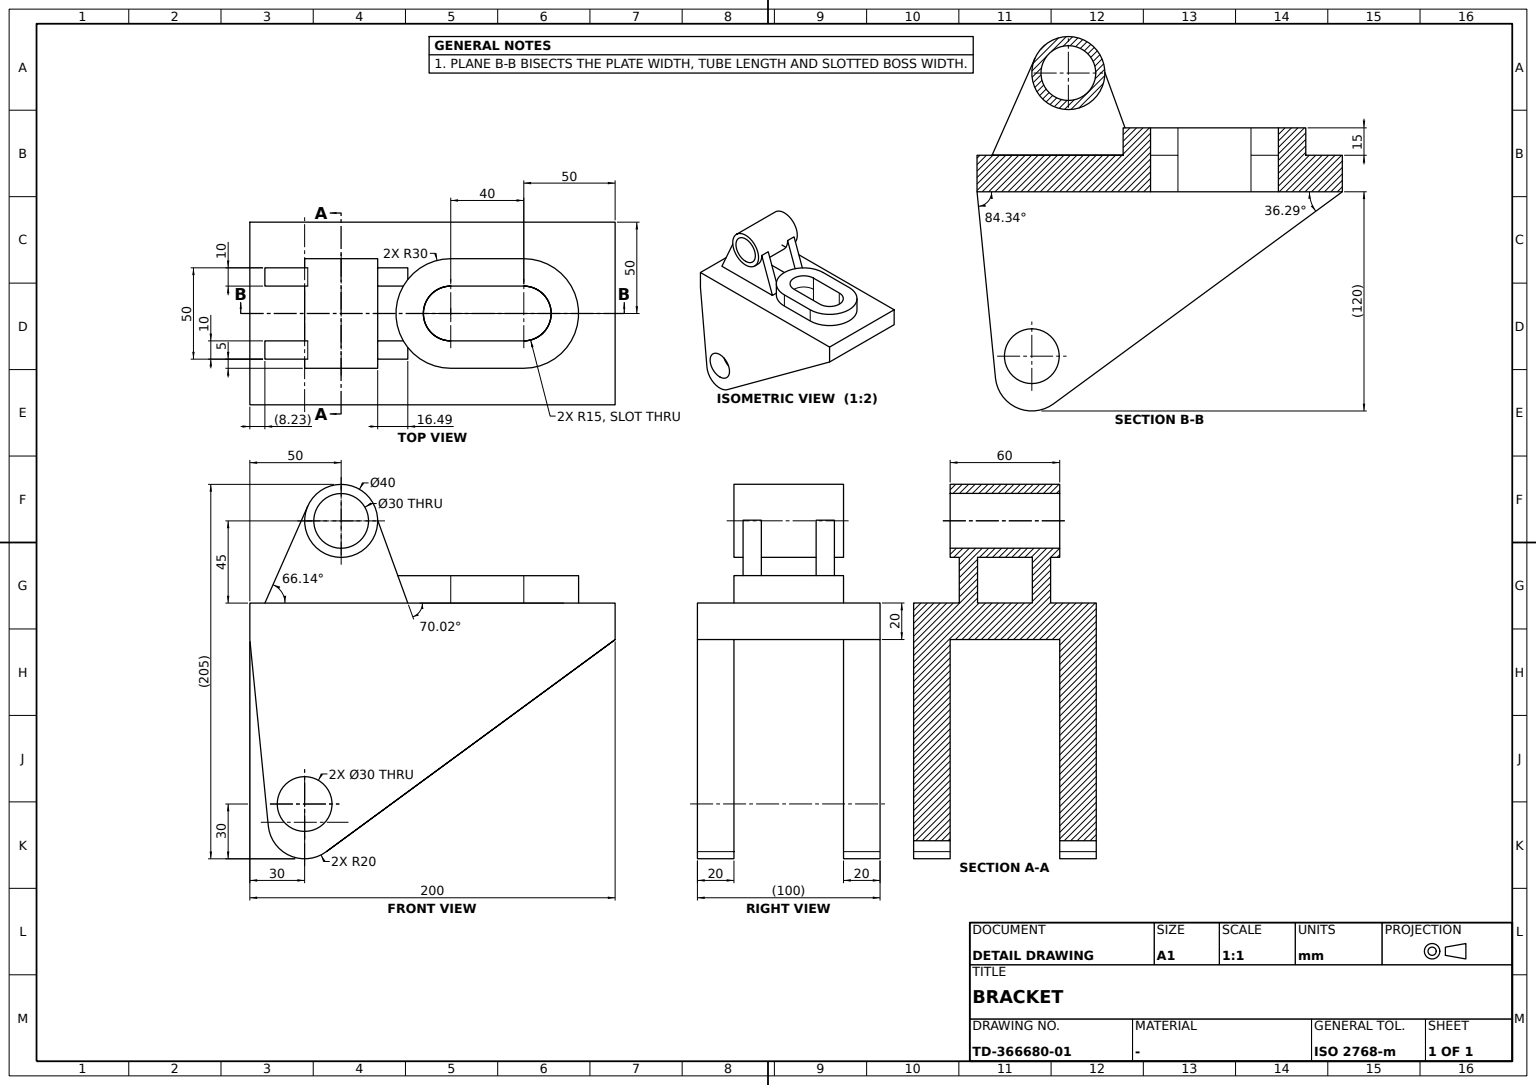
ISO-10303-21;
HEADER;
FILE_DESCRIPTION((''),'2;1');
FILE_NAME('','',(''),(''),'','','');
FILE_SCHEMA(('AUTOMOTIVE_DESIGN'));
ENDSEC;
DATA;
#1=APPLICATION_CONTEXT('');
#2=PRODUCT_CONTEXT('',#1,'mechanical');
#3=PRODUCT('','','',(#2));
#4=PRODUCT_DEFINITION_FORMATION('','',#3);
#5=PRODUCT_DEFINITION_CONTEXT('',#1,'design');
#6=PRODUCT_DEFINITION('','',#4,#5);
#7=PRODUCT_DEFINITION_SHAPE('','',#6);
#8=(LENGTH_UNIT()NAMED_UNIT(*)SI_UNIT(.MILLI.,.METRE.));
#9=(NAMED_UNIT(*)PLANE_ANGLE_UNIT()SI_UNIT($,.RADIAN.));
#10=(NAMED_UNIT(*)SI_UNIT($,.STERADIAN.)SOLID_ANGLE_UNIT());
#11=UNCERTAINTY_MEASURE_WITH_UNIT(LENGTH_MEASURE(0.005),#8,'distance_accuracy_value','');
#12=(GEOMETRIC_REPRESENTATION_CONTEXT(3)GLOBAL_UNCERTAINTY_ASSIGNED_CONTEXT((#11))GLOBAL_UNIT_ASSIGNED_CONTEXT((#8,#9,#10))REPRESENTATION_CONTEXT('',''));
#13=CARTESIAN_POINT('',(-48.163796,-50.,-136.121547));
#14=VERTEX_POINT('',#13);
#15=CARTESIAN_POINT('',(-48.163796,-30.,-136.121547));
#16=VERTEX_POINT('',#15);
#17=CARTESIAN_POINT('',(-48.163796,-40.,-136.121547));
#18=DIRECTION('',(0.,-1.,0.));
#19=VECTOR('',#18,1000.);
#20=LINE('',#17,#19);
#21=EDGE_CURVE('',#14,#16,#20,.F.);
#22=ORIENTED_EDGE('',*,*,#21,.F.);
#23=CARTESIAN_POINT('',(-79.902662,-50.,-121.970799));
#24=VERTEX_POINT('',#23);
#25=CARTESIAN_POINT('',(-60.,-50.,-120.));
#26=DIRECTION('',(0.,0.,-1.));
#27=AXIS2_PLACEMENT_3D('',#25,#18,#26);
#28=CIRCLE('',#27,20.);
#29=EDGE_CURVE('',#24,#14,#28,.T.);
#30=ORIENTED_EDGE('',*,*,#29,.F.);
#31=CARTESIAN_POINT('',(-79.902662,-30.,-121.970799));
#32=VERTEX_POINT('',#31);
#33=CARTESIAN_POINT('',(-79.902662,-40.,-121.970799));
#34=LINE('',#33,#19);
#35=EDGE_CURVE('',#24,#32,#34,.F.);
#36=ORIENTED_EDGE('',*,*,#35,.T.);
#37=CARTESIAN_POINT('',(-60.,-30.,-120.));
#38=AXIS2_PLACEMENT_3D('',#37,#18,#26);
#39=CIRCLE('',#38,20.);
#40=EDGE_CURVE('',#32,#16,#39,.T.);
#41=ORIENTED_EDGE('',*,*,#40,.T.);
#42=EDGE_LOOP('',(#22,#30,#36,#41));
#43=FACE_BOUND('',#42,.T.);
#44=CARTESIAN_POINT('',(-60.,-40.,-120.));
#45=DIRECTION('',(1.,0.,0.));
#46=AXIS2_PLACEMENT_3D('',#44,#18,#45);
#47=CYLINDRICAL_SURFACE('',#46,20.);
#48=ADVANCED_FACE('',(#43),#47,.T.);
#49=CARTESIAN_POINT('',(-5.980762,15.,6.781153));
#50=VERTEX_POINT('',#49);
#51=CARTESIAN_POINT('',(-20.002914,15.,45.34137));
#52=VERTEX_POINT('',#51);
#53=CARTESIAN_POINT('',(-3.514844,15.,0.));
#54=DIRECTION('',(-0.341748537,0.,0.939791433));
#55=VECTOR('',#54,1000.);
#56=LINE('',#53,#55);
#57=EDGE_CURVE('',#50,#52,#56,.T.);
#58=ORIENTED_EDGE('',*,*,#57,.F.);
#59=CARTESIAN_POINT('',(-3.514844,18.629335,0.));
#60=VERTEX_POINT('',#59);
#61=CARTESIAN_POINT('',(20.,0.,-64.664647));
#62=DIRECTION('',(-0.939791433,0.,-0.341748537));
#63=AXIS2_PLACEMENT_3D('',#61,#62,#54);
#64=ELLIPSE('',#63,87.783843,30.);
#65=EDGE_CURVE('',#50,#60,#64,.T.);
#66=ORIENTED_EDGE('',*,*,#65,.T.);
#67=CARTESIAN_POINT('',(-3.514844,25.,0.));
#68=VERTEX_POINT('',#67);
#69=CARTESIAN_POINT('',(-3.514844,0.,0.));
#70=LINE('',#69,#19);
#71=EDGE_CURVE('',#68,#60,#70,.T.);
#72=ORIENTED_EDGE('',*,*,#71,.F.);
#73=CARTESIAN_POINT('',(-20.002914,25.,45.34137));
#74=VERTEX_POINT('',#73);
#75=CARTESIAN_POINT('',(-3.104338,25.,-1.128871));
#76=LINE('',#75,#55);
#77=EDGE_CURVE('',#68,#74,#76,.T.);
#78=ORIENTED_EDGE('',*,*,#77,.T.);
#79=DIRECTION('',(0.,1.,0.));
#80=VECTOR('',#79,1000.);
#81=LINE('',#73,#80);
#82=EDGE_CURVE('',#74,#52,#81,.F.);
#83=ORIENTED_EDGE('',*,*,#82,.T.);
#84=EDGE_LOOP('',(#58,#66,#72,#78,#83));
#85=FACE_BOUND('',#84,.T.);
#86=CARTESIAN_POINT('',(-3.514844,-25.,0.));
#87=AXIS2_PLACEMENT_3D('',#86,#62,#54);
#88=PLANE('',#87);
#89=ADVANCED_FACE('',(#85),#88,.F.);
#90=CARTESIAN_POINT('',(20.,30.,15.));
#91=VERTEX_POINT('',#90);
#92=CARTESIAN_POINT('',(20.,-30.,15.));
#93=VERTEX_POINT('',#92);
#94=CARTESIAN_POINT('',(20.,0.,15.));
#95=DIRECTION('',(0.,0.,1.));
#96=AXIS2_PLACEMENT_3D('',#94,#95,#45);
#97=CIRCLE('',#96,30.);
#98=EDGE_CURVE('',#91,#93,#97,.T.);
#99=ORIENTED_EDGE('',*,*,#98,.F.);
#100=CARTESIAN_POINT('',(20.,30.,0.));
#101=VERTEX_POINT('',#100);
#102=CARTESIAN_POINT('',(20.,30.,7.5));
#103=VECTOR('',#95,1000.);
#104=LINE('',#102,#103);
#105=EDGE_CURVE('',#101,#91,#104,.T.);
#106=ORIENTED_EDGE('',*,*,#105,.F.);
#107=CARTESIAN_POINT('',(20.,0.,0.));
#108=AXIS2_PLACEMENT_3D('',#107,#95,#45);
#109=CIRCLE('',#108,30.);
#110=EDGE_CURVE('',#101,#60,#109,.T.);
#111=ORIENTED_EDGE('',*,*,#110,.T.);
#112=ORIENTED_EDGE('',*,*,#65,.F.);
#113=CARTESIAN_POINT('',(-5.980762,15.,0.));
#114=VERTEX_POINT('',#113);
#115=LINE('',#113,#103);
#116=EDGE_CURVE('',#114,#50,#115,.T.);
#117=ORIENTED_EDGE('',*,*,#116,.F.);
#118=CARTESIAN_POINT('',(-5.980762,-15.,0.));
#119=VERTEX_POINT('',#118);
#120=EDGE_CURVE('',#114,#119,#109,.T.);
#121=ORIENTED_EDGE('',*,*,#120,.T.);
#122=CARTESIAN_POINT('',(-5.980762,-15.,6.781153));
#123=VERTEX_POINT('',#122);
#124=LINE('',#118,#103);
#125=EDGE_CURVE('',#119,#123,#124,.T.);
#126=ORIENTED_EDGE('',*,*,#125,.T.);
#127=CARTESIAN_POINT('',(-3.514844,-18.629335,0.));
#128=VERTEX_POINT('',#127);
#129=EDGE_CURVE('',#123,#128,#64,.F.);
#130=ORIENTED_EDGE('',*,*,#129,.T.);
#131=CARTESIAN_POINT('',(20.,-30.,0.));
#132=VERTEX_POINT('',#131);
#133=EDGE_CURVE('',#128,#132,#109,.T.);
#134=ORIENTED_EDGE('',*,*,#133,.T.);
#135=CARTESIAN_POINT('',(20.,-30.,7.5));
#136=LINE('',#135,#103);
#137=EDGE_CURVE('',#132,#93,#136,.T.);
#138=ORIENTED_EDGE('',*,*,#137,.T.);
#139=EDGE_LOOP('',(#99,#106,#111,#112,#117,#121,#126,#130,#134,#138));
#140=FACE_BOUND('',#139,.T.);
#141=CARTESIAN_POINT('',(20.,0.,7.5));
#142=AXIS2_PLACEMENT_3D('',#141,#95,#45);
#143=CYLINDRICAL_SURFACE('',#142,30.);
#144=ADVANCED_FACE('',(#140),#143,.T.);
#145=CARTESIAN_POINT('',(-60.,30.,-95.));
#146=VERTEX_POINT('',#145);
#147=CARTESIAN_POINT('',(-60.,30.,-110.));
#148=AXIS2_PLACEMENT_3D('',#147,#79,#95);
#149=CIRCLE('',#148,15.);
#150=EDGE_CURVE('',#146,#146,#149,.T.);
#151=ORIENTED_EDGE('',*,*,#150,.T.);
#152=EDGE_LOOP('',(#151));
#153=FACE_BOUND('',#152,.T.);
#154=CARTESIAN_POINT('',(110.,30.,-20.));
#155=VERTEX_POINT('',#154);
#156=CARTESIAN_POINT('',(-90.,30.,-20.));
#157=VERTEX_POINT('',#156);
#158=CARTESIAN_POINT('',(0.,30.,-20.));
#159=DIRECTION('',(-1.,0.,0.));
#160=VECTOR('',#159,1000.);
#161=LINE('',#158,#160);
#162=EDGE_CURVE('',#155,#157,#161,.T.);
#163=ORIENTED_EDGE('',*,*,#162,.T.);
#164=CARTESIAN_POINT('',(-79.902662,30.,-121.970796));
#165=VERTEX_POINT('',#164);
#166=DIRECTION('',(0.098539929,0.,-0.995133098));
#167=VECTOR('',#166,1000.);
#168=LINE('',#156,#167);
#169=EDGE_CURVE('',#157,#165,#168,.T.);
#170=ORIENTED_EDGE('',*,*,#169,.T.);
#171=CARTESIAN_POINT('',(-48.163796,30.,-136.121547));
#172=VERTEX_POINT('',#171);
#173=CARTESIAN_POINT('',(-60.,30.,-120.));
#174=AXIS2_PLACEMENT_3D('',#173,#79,#95);
#175=CIRCLE('',#174,20.);
#176=EDGE_CURVE('',#172,#165,#175,.T.);
#177=ORIENTED_EDGE('',*,*,#176,.F.);
#178=DIRECTION('',(-0.806077344,0.,-0.591810202));
#179=VECTOR('',#178,1000.);
#180=LINE('',#154,#179);
#181=EDGE_CURVE('',#155,#172,#180,.T.);
#182=ORIENTED_EDGE('',*,*,#181,.F.);
#183=EDGE_LOOP('',(#163,#170,#177,#182));
#184=FACE_BOUND('',#183,.T.);
#185=CARTESIAN_POINT('',(0.,30.,0.));
#186=AXIS2_PLACEMENT_3D('',#185,#79,#159);
#187=PLANE('',#186);
#188=ADVANCED_FACE('',(#153,#184),#187,.F.);
#189=CARTESIAN_POINT('',(-58.291095,25.,53.089242));
#190=VERTEX_POINT('',#189);
#191=CARTESIAN_POINT('',(-40.,25.,45.));
#192=AXIS2_PLACEMENT_3D('',#191,#79,#95);
#193=CIRCLE('',#192,20.);
#194=EDGE_CURVE('',#74,#190,#193,.T.);
#195=ORIENTED_EDGE('',*,*,#194,.F.);
#196=ORIENTED_EDGE('',*,*,#77,.F.);
#197=CARTESIAN_POINT('',(-81.769829,25.,0.));
#198=VERTEX_POINT('',#197);
#199=CARTESIAN_POINT('',(0.,25.,0.));
#200=VECTOR('',#45,1000.);
#201=LINE('',#199,#200);
#202=EDGE_CURVE('',#198,#68,#201,.T.);
#203=ORIENTED_EDGE('',*,*,#202,.F.);
#204=CARTESIAN_POINT('',(-68.393135,25.,30.246885));
#205=DIRECTION('',(0.404462119,0.,0.914554752));
#206=VECTOR('',#205,1000.);
#207=LINE('',#204,#206);
#208=EDGE_CURVE('',#198,#190,#207,.T.);
#209=ORIENTED_EDGE('',*,*,#208,.T.);
#210=EDGE_LOOP('',(#195,#196,#203,#209));
#211=FACE_BOUND('',#210,.T.);
#212=AXIS2_PLACEMENT_3D('',#199,#79,#159);
#213=PLANE('',#212);
#214=ADVANCED_FACE('',(#211),#213,.T.);
#215=CARTESIAN_POINT('',(110.,-50.,-20.));
#216=VERTEX_POINT('',#215);
#217=DIRECTION('',(0.806077344,0.,0.591810202));
#218=VECTOR('',#217,1000.);
#219=LINE('',#215,#218);
#220=EDGE_CURVE('',#14,#216,#219,.T.);
#221=ORIENTED_EDGE('',*,*,#220,.F.);
#222=ORIENTED_EDGE('',*,*,#21,.T.);
#223=CARTESIAN_POINT('',(110.,-30.,-20.));
#224=VERTEX_POINT('',#223);
#225=LINE('',#223,#218);
#226=EDGE_CURVE('',#16,#224,#225,.T.);
#227=ORIENTED_EDGE('',*,*,#226,.T.);
#228=LINE('',#215,#80);
#229=EDGE_CURVE('',#216,#224,#228,.T.);
#230=ORIENTED_EDGE('',*,*,#229,.F.);
#231=EDGE_LOOP('',(#221,#222,#227,#230));
#232=FACE_BOUND('',#231,.T.);
#233=CARTESIAN_POINT('',(110.,50.,-20.));
#234=DIRECTION('',(-0.591810202,0.,0.806077344));
#235=AXIS2_PLACEMENT_3D('',#233,#234,#178);
#236=PLANE('',#235);
#237=ADVANCED_FACE('',(#232),#236,.F.);
#238=CARTESIAN_POINT('',(-40.,-30.,25.));
#239=VERTEX_POINT('',#238);
#240=CARTESIAN_POINT('',(-40.,-30.,45.));
#241=AXIS2_PLACEMENT_3D('',#240,#18,#26);
#242=CIRCLE('',#241,20.);
#243=EDGE_CURVE('',#239,#239,#242,.F.);
#244=ORIENTED_EDGE('',*,*,#243,.F.);
#245=EDGE_LOOP('',(#244));
#246=FACE_BOUND('',#245,.T.);
#247=CARTESIAN_POINT('',(-40.,-30.,30.));
#248=VERTEX_POINT('',#247);
#249=CIRCLE('',#241,15.);
#250=EDGE_CURVE('',#248,#248,#249,.F.);
#251=ORIENTED_EDGE('',*,*,#250,.T.);
#252=EDGE_LOOP('',(#251));
#253=FACE_BOUND('',#252,.T.);
#254=CARTESIAN_POINT('',(0.,-30.,0.));
#255=AXIS2_PLACEMENT_3D('',#254,#18,#45);
#256=PLANE('',#255);
#257=ADVANCED_FACE('',(#246,#253),#256,.T.);
#258=CARTESIAN_POINT('',(-81.769829,-25.,0.));
#259=VERTEX_POINT('',#258);
#260=CARTESIAN_POINT('',(-58.291095,-25.,53.089242));
#261=VERTEX_POINT('',#260);
#262=CARTESIAN_POINT('',(-68.393135,-25.,30.246885));
#263=LINE('',#262,#206);
#264=EDGE_CURVE('',#259,#261,#263,.T.);
#265=ORIENTED_EDGE('',*,*,#264,.F.);
#266=VERTEX_POINT('',#86);
#267=CARTESIAN_POINT('',(0.,-25.,0.));
#268=LINE('',#267,#200);
#269=EDGE_CURVE('',#259,#266,#268,.T.);
#270=ORIENTED_EDGE('',*,*,#269,.T.);
#271=CARTESIAN_POINT('',(-20.002914,-25.,45.34137));
#272=VERTEX_POINT('',#271);
#273=CARTESIAN_POINT('',(-3.104338,-25.,-1.128871));
#274=LINE('',#273,#55);
#275=EDGE_CURVE('',#266,#272,#274,.T.);
#276=ORIENTED_EDGE('',*,*,#275,.T.);
#277=CARTESIAN_POINT('',(-40.,-25.,45.));
#278=AXIS2_PLACEMENT_3D('',#277,#79,#95);
#279=CIRCLE('',#278,20.);
#280=EDGE_CURVE('',#272,#261,#279,.T.);
#281=ORIENTED_EDGE('',*,*,#280,.T.);
#282=EDGE_LOOP('',(#265,#270,#276,#281));
#283=FACE_BOUND('',#282,.T.);
#284=AXIS2_PLACEMENT_3D('',#267,#79,#159);
#285=PLANE('',#284);
#286=ADVANCED_FACE('',(#283),#285,.F.);
#287=CARTESIAN_POINT('',(60.,-15.,-20.));
#288=VERTEX_POINT('',#287);
#289=CARTESIAN_POINT('',(20.,-15.,-20.));
#290=VERTEX_POINT('',#289);
#291=CARTESIAN_POINT('',(0.,-15.,-20.));
#292=LINE('',#291,#160);
#293=EDGE_CURVE('',#288,#290,#292,.T.);
#294=ORIENTED_EDGE('',*,*,#293,.F.);
#295=CARTESIAN_POINT('',(60.,15.,-20.));
#296=VERTEX_POINT('',#295);
#297=CARTESIAN_POINT('',(62.356194,15.,-20.));
#298=CARTESIAN_POINT('',(64.712389,14.537362,-20.));
#299=CARTESIAN_POINT('',(66.947305,13.61163,-20.));
#300=CARTESIAN_POINT('',(70.933736,10.933736,-20.));
#301=CARTESIAN_POINT('',(73.61163,6.947305,-20.));
#302=CARTESIAN_POINT('',(74.537362,4.712389,-20.));
#303=CARTESIAN_POINT('',(75.462638,0.,-20.));
#304=CARTESIAN_POINT('',(74.537362,-4.712389,-20.));
#305=CARTESIAN_POINT('',(73.61163,-6.947305,-20.));
#306=CARTESIAN_POINT('',(70.933736,-10.933736,-20.));
#307=CARTESIAN_POINT('',(66.947305,-13.61163,-20.));
#308=CARTESIAN_POINT('',(64.712389,-14.537362,-20.));
#309=CARTESIAN_POINT('',(62.356194,-15.,-20.));
#310=B_SPLINE_CURVE_WITH_KNOTS('',5,(#295,#297,#298,#299,#300,#301,#302,#303,#304,#305,#306,#307,#308,#309,#287),.UNSPECIFIED.,.F.,.F.,(6,3,3,3,6),(0.,0.012,0.024,0.036,0.048),.UNSPECIFIED.);
#311=EDGE_CURVE('',#296,#288,#310,.T.);
#312=ORIENTED_EDGE('',*,*,#311,.F.);
#313=CARTESIAN_POINT('',(20.,15.,-20.));
#314=VERTEX_POINT('',#313);
#315=CARTESIAN_POINT('',(0.,15.,-20.));
#316=LINE('',#315,#200);
#317=EDGE_CURVE('',#314,#296,#316,.T.);
#318=ORIENTED_EDGE('',*,*,#317,.F.);
#319=CARTESIAN_POINT('',(17.643806,-15.,-20.));
#320=CARTESIAN_POINT('',(15.287611,-14.537362,-20.));
#321=CARTESIAN_POINT('',(13.052695,-13.61163,-20.));
#322=CARTESIAN_POINT('',(9.066264,-10.933736,-20.));
#323=CARTESIAN_POINT('',(6.38837,-6.947305,-20.));
#324=CARTESIAN_POINT('',(5.462638,-4.712389,-20.));
#325=CARTESIAN_POINT('',(4.537362,0.,-20.));
#326=CARTESIAN_POINT('',(5.462638,4.712389,-20.));
#327=CARTESIAN_POINT('',(6.38837,6.947305,-20.));
#328=CARTESIAN_POINT('',(9.066264,10.933736,-20.));
#329=CARTESIAN_POINT('',(13.052695,13.61163,-20.));
#330=CARTESIAN_POINT('',(15.287611,14.537362,-20.));
#331=CARTESIAN_POINT('',(17.643806,15.,-20.));
#332=B_SPLINE_CURVE_WITH_KNOTS('',5,(#289,#319,#320,#321,#322,#323,#324,#325,#326,#327,#328,#329,#330,#331,#313),.UNSPECIFIED.,.F.,.F.,(6,3,3,3,6),(0.,0.012,0.024,0.036,0.048),.UNSPECIFIED.);
#333=EDGE_CURVE('',#290,#314,#332,.T.);
#334=ORIENTED_EDGE('',*,*,#333,.F.);
#335=EDGE_LOOP('',(#294,#312,#318,#334));
#336=FACE_BOUND('',#335,.T.);
#337=ORIENTED_EDGE('',*,*,#162,.F.);
#338=EDGE_CURVE('',#224,#155,#228,.T.);
#339=ORIENTED_EDGE('',*,*,#338,.F.);
#340=CARTESIAN_POINT('',(-90.,-30.,-20.));
#341=VERTEX_POINT('',#340);
#342=CARTESIAN_POINT('',(0.,-30.,-20.));
#343=LINE('',#342,#200);
#344=EDGE_CURVE('',#341,#224,#343,.T.);
#345=ORIENTED_EDGE('',*,*,#344,.F.);
#346=CARTESIAN_POINT('',(-90.,50.,-20.));
#347=LINE('',#346,#19);
#348=EDGE_CURVE('',#157,#341,#347,.T.);
#349=ORIENTED_EDGE('',*,*,#348,.F.);
#350=EDGE_LOOP('',(#337,#339,#345,#349));
#351=FACE_BOUND('',#350,.T.);
#352=CARTESIAN_POINT('',(0.,0.,-20.));
#353=AXIS2_PLACEMENT_3D('',#352,#95,#45);
#354=PLANE('',#353);
#355=ADVANCED_FACE('',(#336,#351),#354,.F.);
#356=VERTEX_POINT('',#233);
#357=LINE('',#233,#19);
#358=EDGE_CURVE('',#356,#155,#357,.T.);
#359=ORIENTED_EDGE('',*,*,#358,.T.);
#360=ORIENTED_EDGE('',*,*,#181,.T.);
#361=CARTESIAN_POINT('',(-48.163794,50.,-136.121545));
#362=VERTEX_POINT('',#361);
#363=EDGE_CURVE('',#362,#172,#20,.T.);
#364=ORIENTED_EDGE('',*,*,#363,.F.);
#365=LINE('',#233,#179);
#366=EDGE_CURVE('',#356,#362,#365,.T.);
#367=ORIENTED_EDGE('',*,*,#366,.F.);
#368=EDGE_LOOP('',(#359,#360,#364,#367));
#369=FACE_BOUND('',#368,.T.);
#370=ADVANCED_FACE('',(#369),#236,.F.);
#371=CARTESIAN_POINT('',(-60.,-30.,-125.));
#372=VERTEX_POINT('',#371);
#373=CARTESIAN_POINT('',(-60.,-30.,-110.));
#374=AXIS2_PLACEMENT_3D('',#373,#18,#26);
#375=CIRCLE('',#374,15.);
#376=EDGE_CURVE('',#372,#372,#375,.T.);
#377=ORIENTED_EDGE('',*,*,#376,.T.);
#378=EDGE_LOOP('',(#377));
#379=FACE_BOUND('',#378,.T.);
#380=ORIENTED_EDGE('',*,*,#226,.F.);
#381=ORIENTED_EDGE('',*,*,#40,.F.);
#382=CARTESIAN_POINT('',(-91.087296,-30.,-9.019633));
#383=LINE('',#382,#167);
#384=EDGE_CURVE('',#341,#32,#383,.T.);
#385=ORIENTED_EDGE('',*,*,#384,.F.);
#386=ORIENTED_EDGE('',*,*,#344,.T.);
#387=EDGE_LOOP('',(#380,#381,#385,#386));
#388=FACE_BOUND('',#387,.T.);
#389=ADVANCED_FACE('',(#379,#388),#256,.F.);
#390=CARTESIAN_POINT('',(20.,-15.,0.));
#391=VERTEX_POINT('',#390);
#392=LINE('',#390,#103);
#393=EDGE_CURVE('',#391,#290,#392,.F.);
#394=ORIENTED_EDGE('',*,*,#393,.T.);
#395=ORIENTED_EDGE('',*,*,#333,.T.);
#396=CARTESIAN_POINT('',(20.,15.,0.));
#397=VERTEX_POINT('',#396);
#398=LINE('',#396,#103);
#399=EDGE_CURVE('',#397,#314,#398,.F.);
#400=ORIENTED_EDGE('',*,*,#399,.F.);
#401=CARTESIAN_POINT('',(16.073009,-15.,0.));
#402=CARTESIAN_POINT('',(8.250292,-11.754174,0.));
#403=CARTESIAN_POINT('',(3.374854,0.,0.));
#404=CARTESIAN_POINT('',(8.250292,11.754174,0.));
#405=CARTESIAN_POINT('',(16.073009,15.,0.));
#406=B_SPLINE_CURVE_WITH_KNOTS('',3,(#390,#401,#402,#403,#404,#405,#396),.UNSPECIFIED.,.F.,.F.,(4,1,1,1,4),(23.561944902,35.342917353,47.123889804,58.904862255,70.685834706),.UNSPECIFIED.);
#407=EDGE_CURVE('',#397,#391,#406,.F.);
#408=ORIENTED_EDGE('',*,*,#407,.T.);
#409=EDGE_LOOP('',(#394,#395,#400,#408));
#410=FACE_BOUND('',#409,.T.);
#411=CARTESIAN_POINT('',(16.073009,-15.,-20.));
#412=CARTESIAN_POINT('',(8.250292,-11.754174,-20.));
#413=CARTESIAN_POINT('',(3.374854,0.,-20.));
#414=CARTESIAN_POINT('',(8.250292,11.754174,-20.));
#415=CARTESIAN_POINT('',(16.073009,15.,-20.));
#416=B_SPLINE_SURFACE_WITH_KNOTS('',3,1,((#390,#289),(#401,#411),(#402,#412),(#403,#413),(#404,#414),(#405,#415),(#396,#313)),.SURF_OF_LINEAR_EXTRUSION.,.F.,.F.,.F.,(4,1,1,1,4),(2,2),(0.,0.012,0.024,0.036,0.048),(0.,1.),.UNSPECIFIED.);
#417=ADVANCED_FACE('',(#410),#416,.F.);
#418=ORIENTED_EDGE('',*,*,#243,.T.);
#419=EDGE_LOOP('',(#418));
#420=FACE_BOUND('',#419,.T.);
#421=CARTESIAN_POINT('',(-40.,30.,65.));
#422=VERTEX_POINT('',#421);
#423=CARTESIAN_POINT('',(-40.,30.,45.));
#424=AXIS2_PLACEMENT_3D('',#423,#79,#95);
#425=CIRCLE('',#424,20.);
#426=EDGE_CURVE('',#422,#422,#425,.T.);
#427=ORIENTED_EDGE('',*,*,#426,.F.);
#428=EDGE_LOOP('',(#427));
#429=FACE_BOUND('',#428,.T.);
#430=ORIENTED_EDGE('',*,*,#280,.F.);
#431=CARTESIAN_POINT('',(-20.002914,-15.,45.34137));
#432=VERTEX_POINT('',#431);
#433=LINE('',#271,#80);
#434=EDGE_CURVE('',#272,#432,#433,.T.);
#435=ORIENTED_EDGE('',*,*,#434,.T.);
#436=CARTESIAN_POINT('',(-58.291095,-15.,53.089242));
#437=VERTEX_POINT('',#436);
#438=CARTESIAN_POINT('',(-40.,-15.,45.));
#439=AXIS2_PLACEMENT_3D('',#438,#79,#95);
#440=CIRCLE('',#439,20.);
#441=EDGE_CURVE('',#432,#437,#440,.T.);
#442=ORIENTED_EDGE('',*,*,#441,.T.);
#443=CARTESIAN_POINT('',(-58.291095,0.,53.089242));
#444=LINE('',#443,#80);
#445=EDGE_CURVE('',#261,#437,#444,.T.);
#446=ORIENTED_EDGE('',*,*,#445,.F.);
#447=EDGE_LOOP('',(#430,#435,#442,#446));
#448=FACE_BOUND('',#447,.T.);
#449=ORIENTED_EDGE('',*,*,#194,.T.);
#450=CARTESIAN_POINT('',(-58.291095,15.,53.089242));
#451=VERTEX_POINT('',#450);
#452=EDGE_CURVE('',#190,#451,#444,.F.);
#453=ORIENTED_EDGE('',*,*,#452,.T.);
#454=CARTESIAN_POINT('',(-40.,15.,45.));
#455=AXIS2_PLACEMENT_3D('',#454,#18,#26);
#456=CIRCLE('',#455,20.);
#457=EDGE_CURVE('',#451,#52,#456,.T.);
#458=ORIENTED_EDGE('',*,*,#457,.T.);
#459=ORIENTED_EDGE('',*,*,#82,.F.);
#460=EDGE_LOOP('',(#449,#453,#458,#459));
#461=FACE_BOUND('',#460,.T.);
#462=CARTESIAN_POINT('',(-40.,0.,45.));
#463=AXIS2_PLACEMENT_3D('',#462,#79,#159);
#464=CYLINDRICAL_SURFACE('',#463,20.);
#465=ADVANCED_FACE('',(#420,#429,#448,#461),#464,.T.);
#466=VERTEX_POINT('',#346);
#467=EDGE_CURVE('',#466,#157,#347,.T.);
#468=ORIENTED_EDGE('',*,*,#467,.F.);
#469=CARTESIAN_POINT('',(-79.902662,50.,-121.970799));
#470=VERTEX_POINT('',#469);
#471=LINE('',#346,#167);
#472=EDGE_CURVE('',#466,#470,#471,.T.);
#473=ORIENTED_EDGE('',*,*,#472,.T.);
#474=EDGE_CURVE('',#470,#165,#34,.T.);
#475=ORIENTED_EDGE('',*,*,#474,.T.);
#476=ORIENTED_EDGE('',*,*,#169,.F.);
#477=EDGE_LOOP('',(#468,#473,#475,#476));
#478=FACE_BOUND('',#477,.T.);
#479=DIRECTION('',(-0.995133098,0.,-0.098539929));
#480=AXIS2_PLACEMENT_3D('',#346,#479,#166);
#481=PLANE('',#480);
#482=ADVANCED_FACE('',(#478),#481,.T.);
#483=CARTESIAN_POINT('',(-60.,50.,-95.));
#484=VERTEX_POINT('',#483);
#485=CARTESIAN_POINT('',(-60.,50.,-110.));
#486=AXIS2_PLACEMENT_3D('',#485,#79,#95);
#487=CIRCLE('',#486,15.);
#488=EDGE_CURVE('',#484,#484,#487,.T.);
#489=ORIENTED_EDGE('',*,*,#488,.T.);
#490=EDGE_LOOP('',(#489));
#491=FACE_BOUND('',#490,.T.);
#492=ORIENTED_EDGE('',*,*,#150,.F.);
#493=EDGE_LOOP('',(#492));
#494=FACE_BOUND('',#493,.T.);
#495=CARTESIAN_POINT('',(-60.,-0.66,-110.));
#496=AXIS2_PLACEMENT_3D('',#495,#79,#159);
#497=CYLINDRICAL_SURFACE('',#496,15.);
#498=ADVANCED_FACE('',(#491,#494),#497,.F.);
#499=CARTESIAN_POINT('',(60.,30.,0.));
#500=VERTEX_POINT('',#499);
#501=LINE('',#185,#200);
#502=EDGE_CURVE('',#101,#500,#501,.T.);
#503=ORIENTED_EDGE('',*,*,#502,.F.);
#504=ORIENTED_EDGE('',*,*,#105,.T.);
#505=CARTESIAN_POINT('',(60.,30.,15.));
#506=VERTEX_POINT('',#505);
#507=CARTESIAN_POINT('',(0.,30.,15.));
#508=LINE('',#507,#200);
#509=EDGE_CURVE('',#91,#506,#508,.T.);
#510=ORIENTED_EDGE('',*,*,#509,.T.);
#511=CARTESIAN_POINT('',(60.,30.,7.5));
#512=LINE('',#511,#103);
#513=EDGE_CURVE('',#500,#506,#512,.T.);
#514=ORIENTED_EDGE('',*,*,#513,.F.);
#515=EDGE_LOOP('',(#503,#504,#510,#514));
#516=FACE_BOUND('',#515,.T.);
#517=ADVANCED_FACE('',(#516),#187,.T.);
#518=CARTESIAN_POINT('',(60.,-15.,15.));
#519=VERTEX_POINT('',#518);
#520=CARTESIAN_POINT('',(60.,15.,15.));
#521=VERTEX_POINT('',#520);
#522=CARTESIAN_POINT('',(60.,0.,15.));
#523=AXIS2_PLACEMENT_3D('',#522,#95,#45);
#524=CIRCLE('',#523,15.);
#525=EDGE_CURVE('',#519,#521,#524,.T.);
#526=ORIENTED_EDGE('',*,*,#525,.T.);
#527=CARTESIAN_POINT('',(60.,15.,0.));
#528=VERTEX_POINT('',#527);
#529=CARTESIAN_POINT('',(60.,15.,7.5));
#530=LINE('',#529,#103);
#531=EDGE_CURVE('',#528,#521,#530,.T.);
#532=ORIENTED_EDGE('',*,*,#531,.F.);
#533=CARTESIAN_POINT('',(60.,-15.,0.));
#534=VERTEX_POINT('',#533);
#535=CARTESIAN_POINT('',(63.926991,15.,0.));
#536=CARTESIAN_POINT('',(71.749708,11.754174,0.));
#537=CARTESIAN_POINT('',(76.625146,0.,0.));
#538=CARTESIAN_POINT('',(71.749708,-11.754174,0.));
#539=CARTESIAN_POINT('',(63.926991,-15.,0.));
#540=B_SPLINE_CURVE_WITH_KNOTS('',3,(#527,#535,#536,#537,#538,#539,#533),.UNSPECIFIED.,.F.,.F.,(4,1,1,1,4),(70.685834706,82.466807157,94.247779608,106.028752059,117.80972451),.UNSPECIFIED.);
#541=EDGE_CURVE('',#528,#534,#540,.T.);
#542=ORIENTED_EDGE('',*,*,#541,.T.);
#543=CARTESIAN_POINT('',(60.,-15.,7.5));
#544=LINE('',#543,#103);
#545=EDGE_CURVE('',#534,#519,#544,.T.);
#546=ORIENTED_EDGE('',*,*,#545,.T.);
#547=EDGE_LOOP('',(#526,#532,#542,#546));
#548=FACE_BOUND('',#547,.T.);
#549=CARTESIAN_POINT('',(60.,0.,7.5));
#550=AXIS2_PLACEMENT_3D('',#549,#95,#45);
#551=CYLINDRICAL_SURFACE('',#550,15.);
#552=ADVANCED_FACE('',(#548),#551,.F.);
#553=ORIENTED_EDGE('',*,*,#317,.T.);
#554=LINE('',#527,#103);
#555=EDGE_CURVE('',#528,#296,#554,.F.);
#556=ORIENTED_EDGE('',*,*,#555,.F.);
#557=ORIENTED_EDGE('',*,*,#531,.T.);
#558=CARTESIAN_POINT('',(20.,15.,15.));
#559=VERTEX_POINT('',#558);
#560=CARTESIAN_POINT('',(0.,15.,15.));
#561=LINE('',#560,#200);
#562=EDGE_CURVE('',#559,#521,#561,.T.);
#563=ORIENTED_EDGE('',*,*,#562,.F.);
#564=CARTESIAN_POINT('',(20.,15.,7.5));
#565=LINE('',#564,#103);
#566=EDGE_CURVE('',#397,#559,#565,.T.);
#567=ORIENTED_EDGE('',*,*,#566,.F.);
#568=ORIENTED_EDGE('',*,*,#399,.T.);
#569=EDGE_LOOP('',(#553,#556,#557,#563,#567,#568));
#570=FACE_BOUND('',#569,.T.);
#571=AXIS2_PLACEMENT_3D('',#396,#18,#45);
#572=PLANE('',#571);
#573=ADVANCED_FACE('',(#570),#572,.T.);
#574=ORIENTED_EDGE('',*,*,#376,.F.);
#575=EDGE_LOOP('',(#574));
#576=FACE_BOUND('',#575,.T.);
#577=CARTESIAN_POINT('',(-60.,-50.,-125.));
#578=VERTEX_POINT('',#577);
#579=CARTESIAN_POINT('',(-60.,-50.,-110.));
#580=AXIS2_PLACEMENT_3D('',#579,#18,#26);
#581=CIRCLE('',#580,15.);
#582=EDGE_CURVE('',#578,#578,#581,.T.);
#583=ORIENTED_EDGE('',*,*,#582,.T.);
#584=EDGE_LOOP('',(#583));
#585=FACE_BOUND('',#584,.T.);
#586=ADVANCED_FACE('',(#576,#585),#497,.F.);
#587=ORIENTED_EDGE('',*,*,#566,.T.);
#588=CARTESIAN_POINT('',(20.,-15.,15.));
#589=VERTEX_POINT('',#588);
#590=CIRCLE('',#96,15.);
#591=EDGE_CURVE('',#559,#589,#590,.T.);
#592=ORIENTED_EDGE('',*,*,#591,.T.);
#593=CARTESIAN_POINT('',(20.,-15.,7.5));
#594=LINE('',#593,#103);
#595=EDGE_CURVE('',#391,#589,#594,.T.);
#596=ORIENTED_EDGE('',*,*,#595,.F.);
#597=ORIENTED_EDGE('',*,*,#407,.F.);
#598=EDGE_LOOP('',(#587,#592,#596,#597));
#599=FACE_BOUND('',#598,.T.);
#600=CYLINDRICAL_SURFACE('',#142,15.);
#601=ADVANCED_FACE('',(#599),#600,.F.);
#602=ORIENTED_EDGE('',*,*,#98,.T.);
#603=CARTESIAN_POINT('',(60.,-30.,15.));
#604=VERTEX_POINT('',#603);
#605=CARTESIAN_POINT('',(0.,-30.,15.));
#606=LINE('',#605,#160);
#607=EDGE_CURVE('',#604,#93,#606,.T.);
#608=ORIENTED_EDGE('',*,*,#607,.F.);
#609=CIRCLE('',#523,30.);
#610=EDGE_CURVE('',#604,#506,#609,.T.);
#611=ORIENTED_EDGE('',*,*,#610,.T.);
#612=ORIENTED_EDGE('',*,*,#509,.F.);
#613=EDGE_LOOP('',(#602,#608,#611,#612));
#614=FACE_BOUND('',#613,.T.);
#615=ORIENTED_EDGE('',*,*,#591,.F.);
#616=ORIENTED_EDGE('',*,*,#562,.T.);
#617=ORIENTED_EDGE('',*,*,#525,.F.);
#618=CARTESIAN_POINT('',(0.,-15.,15.));
#619=LINE('',#618,#160);
#620=EDGE_CURVE('',#519,#589,#619,.T.);
#621=ORIENTED_EDGE('',*,*,#620,.T.);
#622=EDGE_LOOP('',(#615,#616,#617,#621));
#623=FACE_BOUND('',#622,.T.);
#624=CARTESIAN_POINT('',(0.,0.,15.));
#625=AXIS2_PLACEMENT_3D('',#624,#95,#45);
#626=PLANE('',#625);
#627=ADVANCED_FACE('',(#614,#623),#626,.T.);
#628=CARTESIAN_POINT('',(-60.,50.,-120.));
#629=AXIS2_PLACEMENT_3D('',#628,#79,#95);
#630=CIRCLE('',#629,20.);
#631=EDGE_CURVE('',#362,#470,#630,.T.);
#632=ORIENTED_EDGE('',*,*,#631,.F.);
#633=ORIENTED_EDGE('',*,*,#363,.T.);
#634=ORIENTED_EDGE('',*,*,#176,.T.);
#635=ORIENTED_EDGE('',*,*,#474,.F.);
#636=EDGE_LOOP('',(#632,#633,#634,#635));
#637=FACE_BOUND('',#636,.T.);
#638=ADVANCED_FACE('',(#637),#47,.T.);
#639=CARTESIAN_POINT('',(-81.769829,-15.,0.));
#640=VERTEX_POINT('',#639);
#641=LINE('',#533,#200);
#642=EDGE_CURVE('',#640,#119,#641,.T.);
#643=ORIENTED_EDGE('',*,*,#642,.T.);
#644=ORIENTED_EDGE('',*,*,#120,.F.);
#645=CARTESIAN_POINT('',(-81.769829,15.,0.));
#646=VERTEX_POINT('',#645);
#647=CARTESIAN_POINT('',(0.,15.,0.));
#648=LINE('',#647,#200);
#649=EDGE_CURVE('',#646,#114,#648,.T.);
#650=ORIENTED_EDGE('',*,*,#649,.F.);
#651=CARTESIAN_POINT('',(-81.769829,0.,0.));
#652=LINE('',#651,#19);
#653=EDGE_CURVE('',#198,#646,#652,.T.);
#654=ORIENTED_EDGE('',*,*,#653,.F.);
#655=ORIENTED_EDGE('',*,*,#202,.T.);
#656=ORIENTED_EDGE('',*,*,#71,.T.);
#657=ORIENTED_EDGE('',*,*,#110,.F.);
#658=ORIENTED_EDGE('',*,*,#502,.T.);
#659=CARTESIAN_POINT('',(60.,-30.,0.));
#660=VERTEX_POINT('',#659);
#661=CARTESIAN_POINT('',(60.,0.,0.));
#662=AXIS2_PLACEMENT_3D('',#661,#95,#45);
#663=CIRCLE('',#662,30.);
#664=EDGE_CURVE('',#660,#500,#663,.T.);
#665=ORIENTED_EDGE('',*,*,#664,.F.);
#666=LINE('',#254,#160);
#667=EDGE_CURVE('',#660,#132,#666,.T.);
#668=ORIENTED_EDGE('',*,*,#667,.T.);
#669=ORIENTED_EDGE('',*,*,#133,.F.);
#670=LINE('',#86,#80);
#671=EDGE_CURVE('',#266,#128,#670,.T.);
#672=ORIENTED_EDGE('',*,*,#671,.F.);
#673=ORIENTED_EDGE('',*,*,#269,.F.);
#674=LINE('',#258,#80);
#675=EDGE_CURVE('',#259,#640,#674,.T.);
#676=ORIENTED_EDGE('',*,*,#675,.T.);
#677=EDGE_LOOP('',(#643,#644,#650,#654,#655,#656,#657,#658,#665,#668,#669,#672,#673,#676));
#678=FACE_BOUND('',#677,.T.);
#679=CARTESIAN_POINT('',(110.,-50.,0.));
#680=VERTEX_POINT('',#679);
#681=CARTESIAN_POINT('',(110.,50.,0.));
#682=VERTEX_POINT('',#681);
#683=LINE('',#679,#80);
#684=EDGE_CURVE('',#680,#682,#683,.T.);
#685=ORIENTED_EDGE('',*,*,#684,.T.);
#686=CARTESIAN_POINT('',(-90.,50.,0.));
#687=VERTEX_POINT('',#686);
#688=LINE('',#686,#200);
#689=EDGE_CURVE('',#687,#682,#688,.T.);
#690=ORIENTED_EDGE('',*,*,#689,.F.);
#691=CARTESIAN_POINT('',(-90.,-50.,0.));
#692=VERTEX_POINT('',#691);
#693=LINE('',#686,#19);
#694=EDGE_CURVE('',#687,#692,#693,.T.);
#695=ORIENTED_EDGE('',*,*,#694,.T.);
#696=LINE('',#679,#160);
#697=EDGE_CURVE('',#680,#692,#696,.T.);
#698=ORIENTED_EDGE('',*,*,#697,.F.);
#699=EDGE_LOOP('',(#685,#690,#695,#698));
#700=FACE_BOUND('',#699,.T.);
#701=CARTESIAN_POINT('',(0.,0.,0.));
#702=AXIS2_PLACEMENT_3D('',#701,#95,#45);
#703=PLANE('',#702);
#704=ADVANCED_FACE('',(#678,#700),#703,.T.);
#705=ORIENTED_EDGE('',*,*,#434,.F.);
#706=ORIENTED_EDGE('',*,*,#275,.F.);
#707=ORIENTED_EDGE('',*,*,#671,.T.);
#708=ORIENTED_EDGE('',*,*,#129,.F.);
#709=CARTESIAN_POINT('',(3.903186,-15.,-20.399211));
#710=LINE('',#709,#55);
#711=EDGE_CURVE('',#123,#432,#710,.T.);
#712=ORIENTED_EDGE('',*,*,#711,.T.);
#713=EDGE_LOOP('',(#705,#706,#707,#708,#712));
#714=FACE_BOUND('',#713,.T.);
#715=ADVANCED_FACE('',(#714),#88,.F.);
#716=ORIENTED_EDGE('',*,*,#582,.F.);
#717=EDGE_LOOP('',(#716));
#718=FACE_BOUND('',#717,.T.);
#719=CARTESIAN_POINT('',(-90.,-50.,-20.));
#720=VERTEX_POINT('',#719);
#721=CARTESIAN_POINT('',(-90.019183,-50.,-19.806271));
#722=LINE('',#721,#167);
#723=EDGE_CURVE('',#720,#24,#722,.T.);
#724=ORIENTED_EDGE('',*,*,#723,.T.);
#725=ORIENTED_EDGE('',*,*,#29,.T.);
#726=ORIENTED_EDGE('',*,*,#220,.T.);
#727=VECTOR('',#26,1000.);
#728=LINE('',#679,#727);
#729=EDGE_CURVE('',#680,#216,#728,.T.);
#730=ORIENTED_EDGE('',*,*,#729,.F.);
#731=ORIENTED_EDGE('',*,*,#697,.T.);
#732=LINE('',#691,#727);
#733=EDGE_CURVE('',#692,#720,#732,.T.);
#734=ORIENTED_EDGE('',*,*,#733,.T.);
#735=EDGE_LOOP('',(#724,#725,#726,#730,#731,#734));
#736=FACE_BOUND('',#735,.T.);
#737=AXIS2_PLACEMENT_3D('',#679,#18,#159);
#738=PLANE('',#737);
#739=ADVANCED_FACE('',(#718,#736),#738,.T.);
#740=ORIENTED_EDGE('',*,*,#607,.T.);
#741=ORIENTED_EDGE('',*,*,#137,.F.);
#742=ORIENTED_EDGE('',*,*,#667,.F.);
#743=CARTESIAN_POINT('',(60.,-30.,7.5));
#744=LINE('',#743,#103);
#745=EDGE_CURVE('',#660,#604,#744,.T.);
#746=ORIENTED_EDGE('',*,*,#745,.T.);
#747=EDGE_LOOP('',(#740,#741,#742,#746));
#748=FACE_BOUND('',#747,.T.);
#749=ADVANCED_FACE('',(#748),#256,.T.);
#750=LINE('',#645,#206);
#751=EDGE_CURVE('',#646,#451,#750,.T.);
#752=ORIENTED_EDGE('',*,*,#751,.F.);
#753=ORIENTED_EDGE('',*,*,#649,.T.);
#754=ORIENTED_EDGE('',*,*,#116,.T.);
#755=ORIENTED_EDGE('',*,*,#57,.T.);
#756=ORIENTED_EDGE('',*,*,#457,.F.);
#757=EDGE_LOOP('',(#752,#753,#754,#755,#756));
#758=FACE_BOUND('',#757,.T.);
#759=ADVANCED_FACE('',(#758),#572,.T.);
#760=ORIENTED_EDGE('',*,*,#384,.T.);
#761=ORIENTED_EDGE('',*,*,#35,.F.);
#762=ORIENTED_EDGE('',*,*,#723,.F.);
#763=LINE('',#346,#80);
#764=EDGE_CURVE('',#720,#341,#763,.T.);
#765=ORIENTED_EDGE('',*,*,#764,.T.);
#766=EDGE_LOOP('',(#760,#761,#762,#765));
#767=FACE_BOUND('',#766,.T.);
#768=ADVANCED_FACE('',(#767),#481,.T.);
#769=ORIENTED_EDGE('',*,*,#751,.T.);
#770=ORIENTED_EDGE('',*,*,#452,.F.);
#771=ORIENTED_EDGE('',*,*,#208,.F.);
#772=ORIENTED_EDGE('',*,*,#653,.T.);
#773=EDGE_LOOP('',(#769,#770,#771,#772));
#774=FACE_BOUND('',#773,.T.);
#775=DIRECTION('',(-0.914554752,0.,0.404462119));
#776=AXIS2_PLACEMENT_3D('',#258,#775,#205);
#777=PLANE('',#776);
#778=ADVANCED_FACE('',(#774),#777,.T.);
#779=ORIENTED_EDGE('',*,*,#711,.F.);
#780=ORIENTED_EDGE('',*,*,#125,.F.);
#781=ORIENTED_EDGE('',*,*,#642,.F.);
#782=CARTESIAN_POINT('',(-58.577758,-15.,52.44105));
#783=LINE('',#782,#206);
#784=EDGE_CURVE('',#640,#437,#783,.T.);
#785=ORIENTED_EDGE('',*,*,#784,.T.);
#786=ORIENTED_EDGE('',*,*,#441,.F.);
#787=EDGE_LOOP('',(#779,#780,#781,#785,#786));
#788=FACE_BOUND('',#787,.T.);
#789=AXIS2_PLACEMENT_3D('',#533,#79,#159);
#790=PLANE('',#789);
#791=ADVANCED_FACE('',(#788),#790,.T.);
#792=ORIENTED_EDGE('',*,*,#620,.F.);
#793=ORIENTED_EDGE('',*,*,#545,.F.);
#794=LINE('',#533,#103);
#795=EDGE_CURVE('',#534,#288,#794,.F.);
#796=ORIENTED_EDGE('',*,*,#795,.T.);
#797=ORIENTED_EDGE('',*,*,#293,.T.);
#798=ORIENTED_EDGE('',*,*,#393,.F.);
#799=ORIENTED_EDGE('',*,*,#595,.T.);
#800=EDGE_LOOP('',(#792,#793,#796,#797,#798,#799));
#801=FACE_BOUND('',#800,.T.);
#802=ADVANCED_FACE('',(#801),#790,.T.);
#803=ORIENTED_EDGE('',*,*,#445,.T.);
#804=ORIENTED_EDGE('',*,*,#784,.F.);
#805=ORIENTED_EDGE('',*,*,#675,.F.);
#806=ORIENTED_EDGE('',*,*,#264,.T.);
#807=EDGE_LOOP('',(#803,#804,#805,#806));
#808=FACE_BOUND('',#807,.T.);
#809=ADVANCED_FACE('',(#808),#777,.T.);
#810=ORIENTED_EDGE('',*,*,#764,.F.);
#811=ORIENTED_EDGE('',*,*,#733,.F.);
#812=ORIENTED_EDGE('',*,*,#694,.F.);
#813=LINE('',#686,#727);
#814=EDGE_CURVE('',#687,#466,#813,.T.);
#815=ORIENTED_EDGE('',*,*,#814,.T.);
#816=ORIENTED_EDGE('',*,*,#467,.T.);
#817=ORIENTED_EDGE('',*,*,#348,.T.);
#818=EDGE_LOOP('',(#810,#811,#812,#815,#816,#817));
#819=FACE_BOUND('',#818,.T.);
#820=AXIS2_PLACEMENT_3D('',#686,#45,#18);
#821=PLANE('',#820);
#822=ADVANCED_FACE('',(#819),#821,.F.);
#823=ORIENTED_EDGE('',*,*,#250,.F.);
#824=EDGE_LOOP('',(#823));
#825=FACE_BOUND('',#824,.T.);
#826=CARTESIAN_POINT('',(-40.,30.,60.));
#827=VERTEX_POINT('',#826);
#828=CIRCLE('',#424,15.);
#829=EDGE_CURVE('',#827,#827,#828,.T.);
#830=ORIENTED_EDGE('',*,*,#829,.T.);
#831=EDGE_LOOP('',(#830));
#832=FACE_BOUND('',#831,.T.);
#833=CYLINDRICAL_SURFACE('',#463,15.);
#834=ADVANCED_FACE('',(#825,#832),#833,.F.);
#835=ORIENTED_EDGE('',*,*,#631,.T.);
#836=ORIENTED_EDGE('',*,*,#472,.F.);
#837=ORIENTED_EDGE('',*,*,#814,.F.);
#838=ORIENTED_EDGE('',*,*,#689,.T.);
#839=LINE('',#681,#727);
#840=EDGE_CURVE('',#682,#356,#839,.T.);
#841=ORIENTED_EDGE('',*,*,#840,.T.);
#842=ORIENTED_EDGE('',*,*,#366,.T.);
#843=EDGE_LOOP('',(#835,#836,#837,#838,#841,#842));
#844=FACE_BOUND('',#843,.T.);
#845=ORIENTED_EDGE('',*,*,#488,.F.);
#846=EDGE_LOOP('',(#845));
#847=FACE_BOUND('',#846,.T.);
#848=AXIS2_PLACEMENT_3D('',#686,#79,#45);
#849=PLANE('',#848);
#850=ADVANCED_FACE('',(#844,#847),#849,.T.);
#851=ORIENTED_EDGE('',*,*,#426,.T.);
#852=EDGE_LOOP('',(#851));
#853=FACE_BOUND('',#852,.T.);
#854=ORIENTED_EDGE('',*,*,#829,.F.);
#855=EDGE_LOOP('',(#854));
#856=FACE_BOUND('',#855,.T.);
#857=ADVANCED_FACE('',(#853,#856),#187,.T.);
#858=ORIENTED_EDGE('',*,*,#555,.T.);
#859=ORIENTED_EDGE('',*,*,#311,.T.);
#860=ORIENTED_EDGE('',*,*,#795,.F.);
#861=ORIENTED_EDGE('',*,*,#541,.F.);
#862=EDGE_LOOP('',(#858,#859,#860,#861));
#863=FACE_BOUND('',#862,.T.);
#864=CARTESIAN_POINT('',(63.926991,15.,-20.));
#865=CARTESIAN_POINT('',(71.749708,11.754174,-20.));
#866=CARTESIAN_POINT('',(76.625146,0.,-20.));
#867=CARTESIAN_POINT('',(71.749708,-11.754174,-20.));
#868=CARTESIAN_POINT('',(63.926991,-15.,-20.));
#869=B_SPLINE_SURFACE_WITH_KNOTS('',3,1,((#527,#295),(#535,#864),(#536,#865),(#537,#866),(#538,#867),(#539,#868),(#533,#287)),.SURF_OF_LINEAR_EXTRUSION.,.F.,.F.,.F.,(4,1,1,1,4),(2,2),(0.,0.012,0.024,0.036,0.048),(0.,1.),.UNSPECIFIED.);
#870=ADVANCED_FACE('',(#863),#869,.F.);
#871=ORIENTED_EDGE('',*,*,#684,.F.);
#872=ORIENTED_EDGE('',*,*,#729,.T.);
#873=ORIENTED_EDGE('',*,*,#229,.T.);
#874=ORIENTED_EDGE('',*,*,#338,.T.);
#875=ORIENTED_EDGE('',*,*,#358,.F.);
#876=ORIENTED_EDGE('',*,*,#840,.F.);
#877=EDGE_LOOP('',(#871,#872,#873,#874,#875,#876));
#878=FACE_BOUND('',#877,.T.);
#879=AXIS2_PLACEMENT_3D('',#679,#159,#79);
#880=PLANE('',#879);
#881=ADVANCED_FACE('',(#878),#880,.F.);
#882=ORIENTED_EDGE('',*,*,#745,.F.);
#883=ORIENTED_EDGE('',*,*,#664,.T.);
#884=ORIENTED_EDGE('',*,*,#513,.T.);
#885=ORIENTED_EDGE('',*,*,#610,.F.);
#886=EDGE_LOOP('',(#882,#883,#884,#885));
#887=FACE_BOUND('',#886,.T.);
#888=CYLINDRICAL_SURFACE('',#550,30.);
#889=ADVANCED_FACE('',(#887),#888,.T.);
#890=CLOSED_SHELL('',(#48,#89,#144,#188,#214,#237,#257,#286,#355,#370,#389,#417,#465,#482,#498,#517,#552,#573,#586,#601,#627,#638,#704,#715,#739,#749,#759,#768,#778,#791,#802,#809,#822,#834,#850,#857,#870,#881,#889));
#891=MANIFOLD_SOLID_BREP('',#890);
#892=ADVANCED_BREP_SHAPE_REPRESENTATION('',(#891),#12);
#893=SHAPE_DEFINITION_REPRESENTATION(#7,#892);
ENDSEC;
END-ISO-10303-21;
